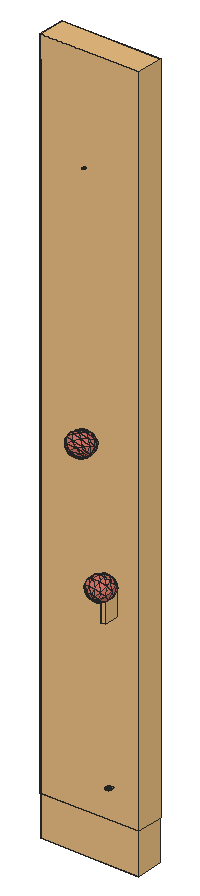
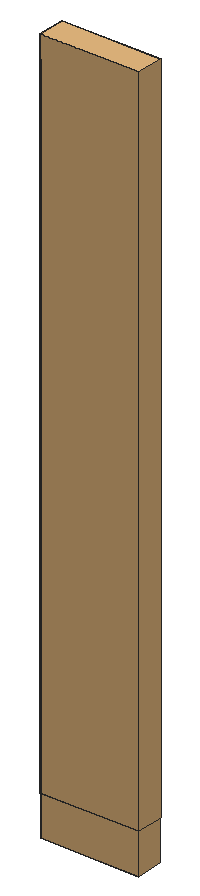
# SketchUp Ruby script. Lengths in inches.
U = 1.inch
M = Sketchup.active_model
def pt(a) = Geom::Point3d.new(a.map { |v| v * U })
def face(e, loops, mat)
  f = e.add_face(loops[0].map { |a| pt(a) })
  loops[1..].each { |l| e.add_face(l.map { |a| pt(a) }).erase! }
  f.material = f.back_material = mat if mat
  f
end
# faces: each face lists its corners as indices into pts; further lists are holes
def faces(e, pts, list, mat = nil) = list.each { |f| face(e, (f[0].is_a?(Array) ? f : [f]).map { |l| l.map { |i| pts[i] } }, mat) }
# xy, xz, yz: faces in a plane at the given z, y or x. An outline is a flat list of corners, or four numbers for a rectangle; further outlines are holes
def ring(l) = l.size == 4 ? [[l[0], l[1]], [l[2], l[1]], [l[2], l[3]], [l[0], l[3]]] : l.each_slice(2).to_a
def flat(e, list, mat, &to3) = list.each { |f| face(e, (f[0].is_a?(Array) ? f : [f]).map { |l| ring(l).map { |u, v| to3.(u, v) } }, mat) }
def xy(e, z, list, mat = nil) = flat(e, list, mat) { |x, y| [x, y, z] }
def xz(e, y, list, mat = nil) = flat(e, list, mat) { |x, z| [x, y, z] }
def yz(e, x, list, mat = nil) = flat(e, list, mat) { |y, z| [x, y, z] }
def lines(e, pts, list) = list.each { |a, b| e.add_line(pt(pts[a]), pt(pts[b])) }
# prism: a flat outline (further loops are holes) pulled along v
def prism(e, loops, v, mat = nil)
  f = face(e, loops, mat); d = Geom::Vector3d.new(v.map { |x| x * U })
  f.pushpull(f.normal.samedirection?(d) ? d.length : -d.length)
end
def box(e, o, s, mat = nil) = prism(e, [[o, [o[0] + s[0], o[1], o[2]], [o[0] + s[0], o[1] + s[1], o[2]], [o[0], o[1] + s[1], o[2]]]], [0, 0, s[2]], mat)
def at(x, y, z, deg = 0) = Geom::Transformation.translation(pt([x, y, z])) * Geom::Transformation.rotation(ORIGIN, Z_AXIS, deg.degrees)
def axes(o, x, y, z) = Geom::Transformation.new([*x, 0, *y, 0, *z, 0, *pt(o).to_a, 1])
def part(name) = M.definitions.add(name)
# library, detail: a bought-in or finely detailed component or shape, given as its bounding box
def library(name, o, s) = part(name).tap { |d| box(d.entities, o, s) }
def detail(e, o, s) = box(e.add_group.entities, o, s)
def put(e, d, t, mat = nil) = e.add_instance(d, t).tap { |i| i.material = mat if mat }
def group(e, t, mat = nil) = e.add_group.tap { |g| g.transformation = t; g.material = mat if mat }.entities
root = M.entities
M.materials.add("green").color = [174, 139, 102]
M.materials.add("vio").color = [206, 114, 100]
c1 = part("3DGeom~237_Defintion")
p = [[47.04,-55.62,-493.71],[-13.56,-317.59,-331.8],[-140.27,-151.99,-445.55],[202.73,-206.32,-387.4],[187.3,88.625,-451.96],[-121.25,109.98,-467.72],
  [-40.27,193.26,-443.62],[-229.4,54.34,-439.92],[-257.06,246.11,-316.41],[364.69,-39.76,-339.2],[242.94,242.09,-331.5],[-8.15,281.87,-374.07],
  [-226.21,-343.77,-187.29],[-324.43,-174.66,-320.41],[-335.72,41.26,-367.67],[202.73,-206.32,-387.4],[116.79,-398.1,-129.14],[-13.56,-317.59,-331.8],
  [202.73,-206.32,-387.4],[304.09,-301.74,-177.3],[364.69,-39.76,-339.2],[304.09,-301.74,-177.3],[202.73,-206.32,-387.4],[-33.49,352.06,-277.72],
  [242.94,242.09,-331.5],[-8.15,281.87,-374.07],[-33.49,352.06,-277.72],[-335.72,41.26,-367.67],[-324.43,-174.66,-320.41],[-456.1,-117.56,-151.8],
  [-335.72,41.26,-367.67],[-411.74,74.22,-270.32],[-335.72,41.26,-367.67],[-257.06,246.11,-316.41],[364.69,-39.76,-339.2],[444.36,-157.49,-135.55],
  [304.09,-301.74,-177.3],[428.9375,137.45,-200.11],[364.69,-39.76,-339.2],[428.9375,137.45,-200.11],[-13.56,-317.59,-331.8],[-67.38,-420.77,-4],
  [-226.21,-343.77,-187.29],[-13.56,-317.59,-331.8],[199.05,363.67,-164.61],[428.9375,137.45,-200.11],[242.94,242.09,-331.5],[-33.49,352.06,-277.72],
  [199.05,363.67,-164.61],[242.94,242.09,-331.5],[-324.43,-174.66,-320.41],[-226.21,-343.77,-187.29],[-378.25,-277.83,7.4],[-324.43,-174.66,-320.41],
  [-437.09,144.42,-173.96],[-257.06,246.11,-316.41],[-404.96,233.02,-104.42],[-257.06,246.11,-316.41],[-323.98,316.3,-80.32],[-257.06,246.11,-316.41],
  [-323.98,316.3,-80.32],[-215.84,371.9375,-108.12],[-257.06,246.11,-316.41],[-109.51,385.02,-180.37],[-33.49,352.06,-277.72],[-257.06,246.11,-316.41],
  [-257.06,246.11,-316.41],[-33.49,352.06,-277.72],[-500,4.02,15.09],[428.9375,137.45,-200.11],[500,-4.02,-15.09],[378.25,277.83,-7.4],
  [428.9375,137.45,-200.11],[199.05,363.67,-164.61],[428.9375,137.45,-200.11],[-226.21,-343.77,-187.29],[-199.05,-363.67,164.61],[-226.21,-343.77,-187.29],
  [-199.05,-363.67,164.61],[-378.25,-277.83,7.4],[67.38,420.77,4],[215.84,-371.9375,108.12],[323.98,-316.3,80.32],[323.98,-316.3,80.32],
  [304.09,-301.74,-177.3],[-444.36,157.49,135.55],[378.25,277.83,-7.4],[-428.9375,-137.45,200.11],[404.96,-233.02,104.42],[323.98,-316.3,80.32],
  [109.51,-385.02,180.37],[-116.78,398.1,129.14],[-304.09,301.73,177.3],[-304.09,301.73,177.3],[-323.98,316.3,-80.32],[-304.09,301.73,177.3],
  [437.09,-144.41,173.96],[456.1,117.56,151.8],[226.21,343.77,187.29],[226.21,343.77,187.29],[378.25,277.83,-7.4],[33.49,-352.06,277.72],
  [-199.05,-363.67,164.61],[-199.05,-363.67,164.61],[-242.94,-242.09,331.5],[-242.94,-242.09,331.5],[-364.69,39.76,339.2],[257.06,-246.11,316.41],
  [323.98,-316.3,80.32],[257.06,-246.11,316.41],[257.06,-246.11,316.41],[13.56,317.59,331.8],[-202.73,206.32,387.4],[-202.73,206.32,387.4],
  [-304.09,301.73,177.3],[411.74,-74.22,270.32],[324.43,174.66,320.41],[226.21,343.77,187.29],[-199.05,-363.67,164.61],[8.15,-281.86,374.07],
  [-242.94,-242.09,331.5],[-199.05,-363.67,164.61],[8.15,-281.86,374.07],[257.06,-246.11,316.41],[-202.73,206.32,387.4],[13.56,317.59,331.8],
  [324.43,174.66,320.41],[226.21,343.77,187.29],[-428.9375,-137.45,200.11],[-242.94,-242.09,331.5],[-187.3,-88.625,451.96],[-428.9375,-137.45,200.11],
  [-364.69,39.76,339.2],[335.72,-41.26,367.67],[257.06,-246.11,316.41],[8.15,-281.86,374.07],[33.49,-352.06,277.72],[257.06,-246.11,316.41],
  [40.27,-193.26,443.62],[257.06,-246.11,316.41],[121.25,-109.98,467.72],[257.06,-246.11,316.41],[229.4,-54.34,439.92],[257.06,-246.11,316.41],
  [335.72,-41.26,367.67],[257.06,-246.11,316.41],[140.27,151.99,445.55],[335.72,-41.26,367.67],[324.43,174.66,320.41],[13.56,317.59,331.8],
  [324.43,174.66,320.41],[-202.73,206.32,387.4],[13.56,317.59,331.8],[-364.69,39.76,339.2],[-47.04,55.62,493.71],[-364.69,39.76,339.2],
  [-202.73,206.32,387.4],[335.72,-41.26,367.67],[-202.73,206.32,387.4]]
faces(c1.entities,p,[[0,1,2],[0,3,1],[4,3,0],[5,0,2],[6,0,5],[6,4,0],[5,2,7],[5,7,8],
  [6,5,8],[4,9,3],[10,9,4],[11,4,6],[11,10,4],[2,12,13],[2,1,12],[7,2,13],
  [11,6,8],[7,13,14],[7,14,8],[15,16,17],[18,19,16],[20,21,22],[23,24,25],[26,11,8],
  [27,28,29],[30,29,31],[32,31,33],[34,35,36],[37,35,38],[10,39,9],[40,41,42],[43,16,41],
  [44,45,46],[47,48,49],[50,51,52],[53,52,29],[31,54,55],[54,56,57],[56,58,59],[60,61,62],
  [63,64,65],[61,63,66],[63,48,67],[31,29,68],[31,68,54],[69,70,35],[71,70,72],[73,71,74],
  [75,41,76],[77,78,79],[63,80,48],[61,80,63],[19,81,16],[19,82,81],[35,83,84],[54,68,85],
  [54,85,56],[80,86,48],[29,52,87],[29,87,68],[35,88,89],[70,88,35],[16,90,41],[16,81,90],
  [60,91,61],[61,91,80],[56,85,92],[56,93,94],[60,95,91],[70,96,88],[97,96,70],[71,97,70],
  [98,97,71],[80,99,100],[41,101,102],[41,90,101],[91,99,80],[52,103,104],[52,105,87],[68,87,106],
  [68,106,85],[81,82,107],[108,88,109],[88,96,110],[90,81,107],[95,111,91],[91,111,99],[85,106,112],
  [85,113,114],[97,115,96],[116,115,97],[117,116,97],[118,119,120],[121,101,122],[96,115,123],[95,124,111],
  [101,90,107],[125,126,127],[128,129,130],[131,130,132],[115,133,134],[116,133,115],[135,136,137],[138,135,139],
  [140,138,141],[142,140,143],[144,142,145],[146,147,148],[149,146,150],[129,135,138],[129,138,130],[151,146,152],
  [153,130,154],[155,154,156],[146,142,157],[158,154,146],[154,140,142],[154,142,146],[130,138,140],[130,140,154]],"vio")
c2 = library("3DGeom~136_Defintion",[-19.91,-529.75,-72.32],[39.82,1000,144.64])
c3 = library("3DGeom~135_Defintion",[-19.41,-483.5625,-70.5],[38.82,1000,141])
c4 = part("3DGeom~46_Defintion")
p = [[-27.13,499.98,25.14],[-34.02,499.92,31.49],[-24.32,499.93,26.43],[-33.96,499.95,29.98],[-34.02,499.92,31.49],[-27.13,499.98,25.14],
  [-33.96,499.95,29.98],[-27.13,499.98,25.14],[-28.64,499.99,25.08],[-31.49,500,26.1],[-33.96,499.95,29.98],[-28.64,499.99,25.08],
  [-27.13,499.98,25.14],[-24.32,499.93,26.43],[-25.67,499.95,25.59],[-31.49,500,26.1],[-28.64,499.99,25.08],[-30.125,500,25.4],
  [-32.66,499.99,27.17],[-33.96,499.95,29.98],[-31.49,500,26.1],[-24.32,499.93,26.43],[-34.02,499.92,31.49],[-22.56,499.86,28.97],
  [-24.32,499.93,26.43],[-22.56,499.86,28.97],[-23.26,499.89,27.6],[-32.66,499.99,27.17],[-33.51,499.97,28.51],[-33.96,499.95,29.98],
  [-22.56,499.86,28.97],[-34.02,499.92,31.49],[-22.29,499.8,31.96],[-22.56,499.86,28.97],[-22.29,499.8,31.96],[-22.23,499.83,30.45],
  [-26.125,499.75,36.54],[-34.02,499.92,31.49],[-29.12,499.77,36.8],[-23.59,499.76,34.77],[-34.02,499.92,31.49],[-26.125,499.75,36.54],
  [-31.92,499.82,35.51],[-34.02,499.92,31.49],[-33.69,499.89,32.97],[-29.12,499.77,36.8],[-34.02,499.92,31.49],[-31.92,499.82,35.51],
  [-22.29,499.8,31.96],[-34.02,499.92,31.49],[-23.59,499.76,34.77],[-22.29,499.8,31.96],[-23.59,499.76,34.77],[-22.74,499.78,33.43],
  [-31.92,499.82,35.51],[-33.69,499.89,32.97],[-32.99,499.85,34.33],[-23.59,499.76,34.77],[-26.125,499.75,36.54],[-24.76,499.75,35.84],
  [-29.12,499.77,36.8],[-31.92,499.82,35.51],[-30.58,499.79,36.35],[-26.125,499.75,36.54],[-29.12,499.77,36.8],[-27.6,499.76,36.86],
  [-53.29,-499.72,58.02],[-51.39,-499.92,55.77],[-50.77,-499.95,55.72],[-53.29,-499.72,58.02],[-50.77,-499.95,55.72],[-53.24,-499.7,58.64],
  [-50.77,-499.95,55.72],[-49.57,-500,56.11],[-53.24,-499.7,58.64],[-50.77,-499.95,55.72],[-50.16,-499.98,55.83],[-49.57,-500,56.11],
  [-52.49,-499.84,56.33],[-51.39,-499.92,55.77],[-53.29,-499.72,58.02],[-52.49,-499.84,56.33],[-51.97,-499.88,55.98],[-51.39,-499.92,55.77],
  [-49.57,-500,56.11],[-48.72,-499.99,57.04],[-53.24,-499.7,58.64],[-49.57,-500,56.11],[-49.08,-500,56.53],[-48.72,-499.99,57.04],
  [-53.29,-499.72,58.02],[-52.91,-499.8,56.82],[-52.49,-499.84,56.33],[-53.29,-499.72,58.02],[-53.18,-499.76,57.41],[-52.91,-499.8,56.82],
  [-48.72,-499.99,57.04],[-48.46,-499.95,58.24],[-53.24,-499.7,58.64],[-48.72,-499.99,57.04],[-48.52,-499.98,57.63],[-48.46,-499.95,58.24],
  [-48.46,-499.95,58.24],[-48.85,-499.875,59.45],[-53.24,-499.7,58.64],[-48.46,-499.95,58.24],[-48.57,-499.91,58.86],[-48.85,-499.875,59.45],
  [-48.85,-499.875,59.45],[-49.78,-499.79,60.29],[-53.24,-499.7,58.64],[-49.78,-499.79,60.29],[-50.98,-499.72,60.54],[-53.24,-499.7,58.64],
  [-52.18,-499.68,60.16],[-53.03,-499.68,59.22],[-53.24,-499.7,58.64],[-50.98,-499.72,60.54],[-52.18,-499.68,60.16],[-53.24,-499.7,58.64],
  [-52.18,-499.68,60.16],[-52.68,-499.67,59.74],[-53.03,-499.68,59.22],[-48.85,-499.875,59.45],[-49.26,-499.83,59.9375],[-49.78,-499.79,60.29],
  [-50.98,-499.72,60.54],[-51.6,-499.69,60.4375],[-52.18,-499.68,60.16],[-49.78,-499.79,60.29],[-50.36,-499.75,60.49],[-50.98,-499.72,60.54]]
faces(c4.entities,p,[[0,1,2],[3,4,5],[6,7,8],[9,10,11],[12,13,14],[15,16,17],[18,19,20],[21,22,23],
  [24,25,26],[27,28,29],[30,31,32],[33,34,35],[36,37,38],[39,40,41],[42,43,44],[45,46,47],
  [48,49,50],[51,52,53],[54,55,56],[57,58,59],[60,61,62],[63,64,65],[66,67,68],[69,70,71],
  [72,73,74],[75,76,77],[78,79,80],[81,82,83],[84,85,86],[87,88,89],[90,91,92],[93,94,95],
  [96,97,98],[99,100,101],[102,103,104],[105,106,107],[108,109,110],[111,112,113],[114,115,116],[117,118,119],
  [120,121,122],[123,124,125],[126,127,128],[129,130,131]],"green")
c5 = part("3DGeom~233_Defintion")
p = [[65.95,-313.47,-334.33],[-179.28,-246.09,-369.2],[-76.8125,-70.73,-489.54],[154.6875,-161.61,-438.54],[-287.73,39.11,-409.37],[46.24,123.59,-478.71],
  [-181.17,207.39,-399.98],[261.25,6.67,-429.16],[261.25,6.67,-429.16],[156.9,284.78,-339.6],[-85.33,346.99,-279.51],[-85.33,346.99,-279.51],
  [156.9,284.78,-339.6],[293.5,-296.87,-209.87],[293.5,-296.87,-209.87],[344.74,-209.1875,-270.04],[344.74,-209.1875,-270.04],[261.25,6.67,-429.16],
  [344.74,-209.1875,-270.04],[261.25,6.67,-429.16],[406.26,-112.03,-264.62],[406.26,-112.03,-264.62],[261.25,6.67,-429.16],[357.09,146.27,-308.69],
  [261.25,6.67,-429.16],[156.9,284.78,-339.6],[357.09,146.27,-308.69],[-376.47,-112.76,-305.15],[-376.47,-112.76,-305.15],[-421.55,138.46,-219.5],
  [-287.73,39.11,-409.37],[-421.55,138.46,-219.5],[-360.03,235.62,-214.08],[-360.03,235.62,-214.08],[-181.17,207.39,-399.98],[-360.03,235.62,-214.08],
  [-304.7,316.22,-144.53],[-181.17,207.39,-399.98],[-85.33,346.99,-279.51],[18.81,-408.24,-144.44],[-233.71,-355.51,-149.9375],[-179.28,-246.09,-369.2],
  [-179.28,-246.09,-369.2],[65.95,-313.47,-334.33],[-233.71,-355.51,-149.9375],[-376.47,-112.76,-305.15],[-179.28,-246.09,-369.2],[156.9,284.78,-339.6],
  [225.52,369.67,-109.5],[156.9,284.78,-339.6],[-25.9,420.5,-80.24],[156.9,284.78,-339.6],[225.52,369.67,-109.5],[266.29,-351.58,-100.24],
  [65.95,-313.47,-334.33],[266.29,-351.58,-100.24],[65.95,-313.47,-334.33],[293.5,-296.87,-209.87],[461.59,-31.43,-195.07],[416.51,219.79,-109.42],
  [-233.71,-355.51,-149.9375],[-423.61,-207.52,-115.26],[-376.47,-112.76,-305.15],[-472.79,50.78,-159.33],[-376.47,-112.76,-305.15],[-376.47,-112.76,-305.15],
  [-421.55,138.46,-219.5],[-270.39,358.66,-29.48],[293.5,-296.87,-209.87],[344.74,-209.1875,-270.04],[442.42,-200.72,-29.18],[-421.55,138.46,-219.5],
  [-442.42,200.72,29.18],[-360.03,235.62,-214.08],[-421.55,138.46,-219.5],[-304.7,316.22,-144.53],[-360.03,235.62,-214.08],[266.29,-351.58,-100.24],
  [495.9,11.01,-80.02],[-500,-3.93,-49.7],[25.9,-420.5,80.24],[-225.52,-369.67,109.5],[-225.52,-369.67,109.5],[-233.71,-355.51,-149.9375],
  [-270.39,358.66,-29.48],[-304.7,316.22,-144.53],[270.39,-358.66,29.48],[270.39,-358.66,29.48],[266.29,-351.58,-100.24],[-225.52,-369.67,109.5],
  [-416.51,-219.79,109.42],[233.71,355.51,149.9375],[225.52,369.67,-109.5],[-18.81,408.24,144.44],[233.71,355.51,149.9375],[225.52,369.67,-109.5],
  [423.61,207.52,115.26],[270.39,-358.66,29.48],[-266.29,351.58,100.24],[500,3.93,49.7],[-495.9,-11.01,80.02],[-266.29,351.58,100.24],
  [-270.39,358.66,-29.48],[304.7,-316.22,144.53],[360.03,-235.62,214.08],[421.55,-138.46,219.5],[472.79,-50.78,159.33],[-461.59,31.43,195.07],
  [-406.26,112.03,264.62],[-344.74,209.1875,270.04],[-344.74,209.1875,270.04],[-293.5,296.87,209.87],[-293.5,296.87,209.87],[-266.29,351.58,100.24],
  [304.7,-316.22,144.53],[270.39,-358.66,29.48],[376.47,112.76,305.15],[-357.09,-146.27,308.69],[85.33,-346.99,279.51],[304.7,-316.22,144.53],
  [-293.5,296.87,209.87],[-156.9,-284.78,339.6],[-225.52,-369.67,109.5],[-156.9,-284.78,339.6],[-156.9,-284.78,339.6],[179.28,246.09,369.2],
  [179.28,246.09,369.2],[-293.5,296.87,209.87],[-65.95,313.47,334.33],[233.71,355.51,149.9375],[-65.95,313.47,334.33],[360.03,-235.62,214.08],
  [304.7,-316.22,144.53],[233.71,355.51,149.9375],[-65.95,313.47,334.33],[179.28,246.09,369.2],[287.73,-39.11,409.37],[287.73,-39.11,409.37],
  [-261.25,-6.67,429.16],[-261.25,-6.67,429.16],[-65.95,313.47,334.33],[-293.5,296.87,209.87],[-344.74,209.1875,270.04],[360.03,-235.62,214.08],
  [181.17,-207.39,399.98],[421.55,-138.46,219.5],[181.17,-207.39,399.98],[360.03,-235.62,214.08],[421.55,-138.46,219.5],[287.73,-39.11,409.37],
  [181.17,-207.39,399.98],[-154.6875,161.61,438.54],[-406.26,112.03,264.62],[-261.25,-6.67,429.16],[-406.26,112.03,264.62],[181.17,-207.39,399.98],
  [-156.9,-284.78,339.6],[85.33,-346.99,279.51],[376.47,112.76,305.15],[76.8125,70.73,489.54],[376.47,112.76,305.15],[179.28,246.09,369.2],
  [-46.24,-123.58,478.71],[-357.09,-146.27,308.69],[-156.9,-284.78,339.6],[-357.09,-146.27,308.69],[181.17,-207.39,399.98],[-156.9,-284.78,339.6],
  [181.17,-207.39,399.98]]
faces(c5.entities,p,[[0,1,2],[0,2,3],[1,4,2],[3,2,5],[2,4,6],[2,6,5],[3,5,7],[8,5,9],
  [5,6,10],[5,11,12],[13,0,3],[14,3,15],[16,3,17],[18,19,20],[21,22,23],[24,25,26],
  [1,27,4],[28,29,30],[4,31,32],[4,33,6],[34,35,36],[37,36,38],[39,40,41],[39,42,43],
  [44,45,46],[23,47,48],[49,38,50],[51,50,52],[53,39,54],[55,56,57],[21,23,58],[58,23,59],
  [23,48,59],[60,61,62],[61,63,64],[65,63,66],[38,36,67],[38,67,50],[68,69,70],[69,21,70],
  [21,58,70],[71,63,72],[73,74,72],[75,76,72],[77,68,70],[58,78,70],[58,59,78],[61,79,63],
  [63,79,72],[80,81,40],[80,40,39],[82,61,83],[84,85,72],[86,80,39],[87,39,88],[89,90,61],
  [90,79,61],[59,48,91],[92,93,94],[95,50,93],[78,59,96],[59,91,96],[97,77,70],[50,67,98],
  [50,98,93],[78,99,70],[78,96,99],[90,100,79],[79,100,72],[101,102,72],[103,97,70],[104,103,70],
  [105,104,70],[106,105,70],[99,106,70],[100,107,72],[107,108,72],[108,109,72],[110,111,72],[112,113,72],
  [114,80,115],[99,116,106],[99,96,116],[117,100,90],[117,107,100],[118,81,80],[119,118,80],[93,98,120],
  [121,90,122],[123,117,90],[118,124,81],[96,125,116],[96,91,126],[93,127,128],[129,93,130],[131,118,132],
  [133,134,135],[106,136,105],[106,116,137],[138,107,117],[139,108,107],[140,141,142],[143,144,118],[145,146,147],
  [148,149,150],[151,152,153],[151,142,154],[140,142,151],[155,156,157],[158,159,149],[160,161,159],[162,163,164],
  [162,153,165],[161,140,151],[166,162,167],[161,151,159],[149,162,168],[149,159,162],[159,153,162],[159,151,153]],"vio")
c6 = library("3DGeom~142_Defintion",[-333.55,-500,-87.71],[667.1,1000,175.42])
c7 = part("3DGeom~143_Defintion")
p = [[307.12,492.85,-37.96],[315.07,468.23,21.32],[327.57,466.68,8.76],[307.12,492.85,-37.96],[327.57,466.68,8.76],[333.55,469.6,-7.65],
  [307.12,492.85,-37.96],[299.4,473.83,26.65],[315.07,468.23,21.32],[307.12,492.85,-37.96],[333.55,469.6,-7.65],[331.42,476.19,-23.54],
  [307.12,492.85,-37.96],[284.77,481.97,23.32],[299.4,473.83,26.65],[307.12,492.85,-37.96],[331.42,476.19,-23.54],[321.75,484.71,-34.63],
  [307.12,492.85,-37.96],[275.09,490.49,12.23],[284.77,481.97,23.32],[307.12,492.85,-37.96],[272.96,497.08,-3.66],[275.09,490.49,12.23],
  [307.12,492.85,-37.96],[278.95,500,-20.08],[272.96,497.08,-3.66],[307.12,492.85,-37.96],[291.45,498.45,-32.63],[278.95,500,-20.08],
  [-307.72,-489.79,19.99],[-291.97,-496.19,23.52],[-279.25,-499.93,35.1875],[-274.79,-496.39,69.05],[-307.72,-489.79,19.99],[-279.25,-499.93,35.1875],
  [-298.8,-482.72,87.71],[-307.72,-489.79,19.99],[-274.79,-496.39,69.05],[-331.73,-476.12,38.65],[-307.72,-489.79,19.99],[-327.27,-472.59,72.51],
  [-307.72,-489.79,19.99],[-331.73,-476.12,38.65],[-322.27,-482.45,25.52],[-327.27,-472.59,72.51],[-307.72,-489.79,19.99],[-298.8,-482.72,87.71],
  [-274.79,-496.39,69.05],[-279.25,-499.93,35.1875],[-272.96,-500,51.85],[-331.73,-476.12,38.65],[-327.27,-472.59,72.51],[-333.55,-472.51,55.85],
  [-298.8,-482.72,87.71],[-274.79,-496.39,69.05],[-284.25,-490.06,82.18],[-327.27,-472.59,72.51],[-298.8,-482.72,87.71],[-314.54,-476.32,84.17]]
faces(c7.entities,p,[[0,1,2],[3,4,5],[6,7,8],[9,10,11],[12,13,14],[15,16,17],[18,19,20],[21,22,23],
  [24,25,26],[27,28,29],[30,31,32],[33,34,35],[36,37,38],[39,40,41],[42,43,44],[45,46,47],
  [48,49,50],[51,52,53],[54,55,56],[57,58,59]],"green")
g1 = group(root,at(15.3125,38.42,26.21))
put(g1,c1,axes([-1.55,0.1875,9.07],[0,0.00039,0],[0,0,-0.00039],[-0.00039,0,0]),"vio")
put(root,c2,axes([13.77,38.96,35.07],[0,0.01014,0],[0,0,-0.01014],[-0.01014,0,0]),"green")
put(root,c3,axes([13.77,38.96,35.07],[0,0.0104,0],[0,0,-0.0104],[-0.0104,0,0]),"green")
put(root,c4,axes([14.37,38.93,34.91],[0,0.00829,0],[0,0,-0.00829],[-0.00829,0,0]),"green")
g2 = group(root,at(15.3125,38.42,26.21))
put(g2,c5,axes([-1.2,0.12,7.3],[0,0.00039,0],[0,0,-0.00039],[-0.00039,0,0]),"vio")
g3 = group(root,at(15.3125,38.42,26.21))
put(g3,c6,axes([-1.17,0.27,7.05],[0,0.00043,0],[0,0,-0.00043],[-0.00043,0,0]),"green")
put(g3,c7,axes([-1.17,0.27,7.05],[0,0.00043,0],[0,0,-0.00043],[-0.00043,0,0]),"green")
